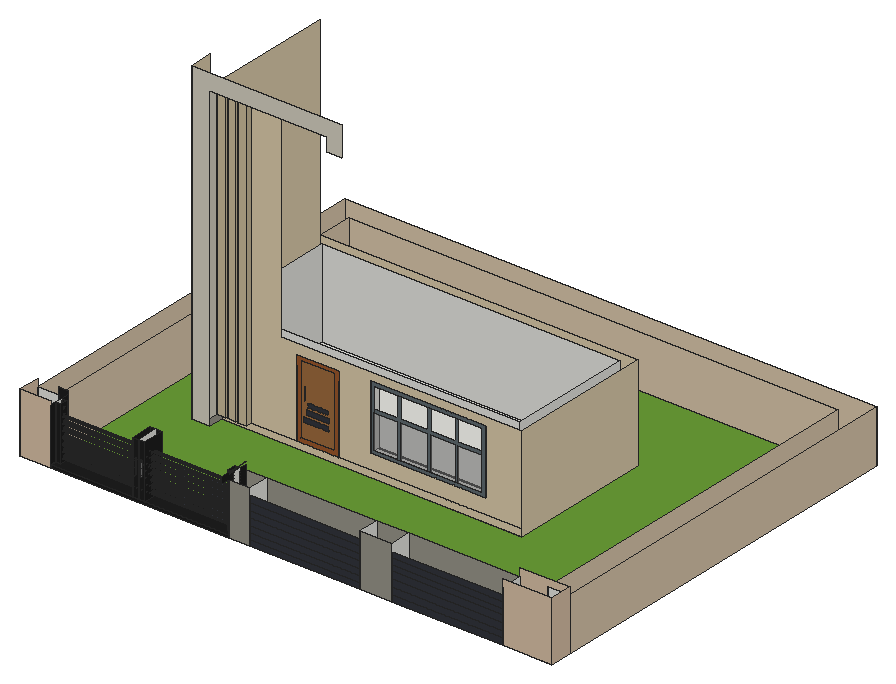
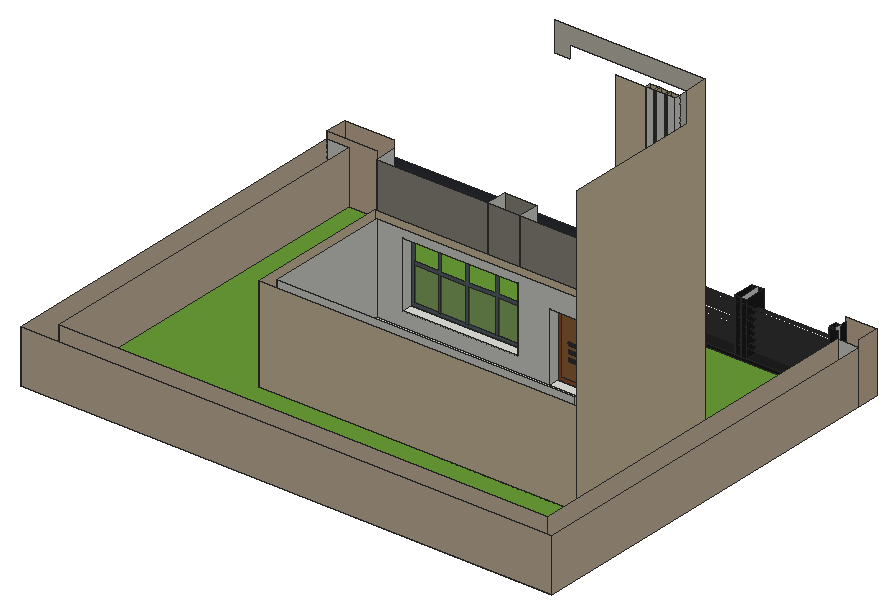
# SketchUp Ruby script. Lengths in inches.
U = 1.inch
M = Sketchup.active_model
def pt(a) = Geom::Point3d.new(a.map { |v| v * U })
def face(e, loops, mat)
  f = e.add_face(loops[0].map { |a| pt(a) })
  loops[1..].each { |l| e.add_face(l.map { |a| pt(a) }).erase! }
  f.material = f.back_material = mat if mat
  f
end
# faces: each face lists its corners as indices into pts; further lists are holes
def faces(e, pts, list, mat = nil) = list.each { |f| face(e, (f[0].is_a?(Array) ? f : [f]).map { |l| l.map { |i| pts[i] } }, mat) }
# xy, xz, yz: faces in a plane at the given z, y or x. An outline is a flat list of corners, or four numbers for a rectangle; further outlines are holes
def ring(l) = l.size == 4 ? [[l[0], l[1]], [l[2], l[1]], [l[2], l[3]], [l[0], l[3]]] : l.each_slice(2).to_a
def flat(e, list, mat, &to3) = list.each { |f| face(e, (f[0].is_a?(Array) ? f : [f]).map { |l| ring(l).map { |u, v| to3.(u, v) } }, mat) }
def xy(e, z, list, mat = nil) = flat(e, list, mat) { |x, y| [x, y, z] }
def xz(e, y, list, mat = nil) = flat(e, list, mat) { |x, z| [x, y, z] }
def yz(e, x, list, mat = nil) = flat(e, list, mat) { |y, z| [x, y, z] }
def lines(e, pts, list) = list.each { |a, b| e.add_line(pt(pts[a]), pt(pts[b])) }
# prism: a flat outline (further loops are holes) pulled along v
def prism(e, loops, v, mat = nil)
  f = face(e, loops, mat); d = Geom::Vector3d.new(v.map { |x| x * U })
  f.pushpull(f.normal.samedirection?(d) ? d.length : -d.length)
end
def box(e, o, s, mat = nil) = prism(e, [[o, [o[0] + s[0], o[1], o[2]], [o[0] + s[0], o[1] + s[1], o[2]], [o[0], o[1] + s[1], o[2]]]], [0, 0, s[2]], mat)
def at(x, y, z, deg = 0) = Geom::Transformation.translation(pt([x, y, z])) * Geom::Transformation.rotation(ORIGIN, Z_AXIS, deg.degrees)
def axes(o, x, y, z) = Geom::Transformation.new([*x, 0, *y, 0, *z, 0, *pt(o).to_a, 1])
def part(name) = M.definitions.add(name)
# library, detail: a bought-in or finely detailed component or shape, given as its bounding box
def library(name, o, s) = part(name).tap { |d| box(d.entities, o, s) }
def detail(e, o, s) = box(e.add_group.entities, o, s)
def put(e, d, t, mat = nil) = e.add_instance(d, t).tap { |i| i.material = mat if mat }
def group(e, t, mat = nil) = e.add_group.tap { |g| g.transformation = t; g.material = mat if mat }.entities
root = M.entities
M.materials.add("[Color M05]").color = [114, 114, 114]
M.materials.add("[Color M08]").color = [30, 30, 30]
M.materials.add("[Field Square Tile]").color = [217, 201, 169]
M.materials.add("[Formica Graystone]").color = [209, 204, 189]
M.materials.add("[Formica Graystone]1").color = [149, 146, 135]
M.materials.add("[Formica Laminate Dark]").color = [50, 53, 60]
M.materials.add("[Formica Laminate Light]").color = [213, 189, 164]
M.materials.add("[Formica Speckled Grey]").color = [94, 105, 111]
M.materials.add("[Grass Dark Green]").color = [106, 157, 55]
M.materials.add("[Quartz Light Brown]").color = [199, 184, 152]
M.materials.add("[Tile Various Tan]").color = [214, 196, 169]
M.materials.add("[Translucent Glass Gray]").color = [128, 128, 128]
M.materials["[Translucent Glass Gray]"].alpha = 0.5
M.materials.add("[Wood Cherry Original]").color = [152, 86, 42]
M.materials.add("[Wood Floor]").color = [155, 105, 61]
xy(root,0,[[0,19.125,41.54,48.44],[41.54,19.125,284.59,48.44],[284.59,19.125,312.84,48.44],[312.84,19.125,463.03,48.44],[463.03,19.125,507.04,48.44],
  [507.04,19.125,658.96,48.44],[658.96,19.125,726.5625,48.44],[0,48.44,0,572.27,726.5625,572.27,726.5625,48.44,697.25,48.44,697.25,542.96,29.31,542.96,29.31,48.44],[92.5625,195.77,92.5625,414.5,526.89,414.5,526.89,216.4,117.23,216.4,117.23,195.77]])
xy(root,0,[[[29.31,48.44,697.25,542.96],[92.5625,195.77,117.23,195.77,117.23,216.4,526.89,216.4,526.89,414.5,92.5625,414.5]]],"[Grass Dark Green]")
xy(root,4.0625,[[153.57,19.125,161.5,48.44],[161.5,19.125,169.43,48.44],[41.54,27.41,48.35,37.79],[277.34,27.41,284.59,37.79]])
xy(root,4.0625,[[41.54,19.125,153.57,19.125,153.57,48.44,41.54,48.44,41.54,37.79,48.35,37.79,48.35,27.41,41.54,27.41],[169.43,19.125,284.59,19.125,284.59,27.41,277.34,27.41,277.34,37.79,284.59,37.79,284.59,48.44,169.43,48.44]],"[Color M08]")
xy(root,9,[[117.23,208.71,128.74,216.4],[131.17,208.71,142.68,216.4],[145.54,208.71,157.05,216.4],[219.375,216.4,276.875,230.18],[106.34,230.18,513.1,400.72]])
xy(root,29.57,[[320.36,216.4,477.43,230.18]])
xz(root,19.125,[[156.51,31.35,159.64,54.1],[163.7,31.35,166.82,54.1]],"[Color M05]")
xz(root,19.125,[[41.54,0,284.59,4.0625],[[153.57,4.0625,161.5,76.75],[156.51,31.35,159.64,54.1]],[[161.5,4.0625,169.43,76.75],[163.7,31.35,166.82,54.1]]],"[Color M08]")
xz(root,19.125,[[284.59,0,312.84,70.6875],[463.03,0,507.04,70.6875]],"[Formica Graystone]1")
xz(root,19.125,[[312.84,0,463.03,7.88],[507.04,0,658.96,8.76],[312.84,7.88,463.03,15.75],[507.04,8.76,658.96,17.52],[312.84,15.75,463.03,24.9375],
  [507.04,17.52,658.96,27.92],[312.84,24.9375,463.03,34.65],[507.04,27.92,658.96,37.26],[312.84,34.65,463.03,42.8],[507.04,37.26,658.96,44.93],
  [312.84,42.8,463.03,52.5625],[507.04,44.93,658.96,53.11],[312.84,52.5625,463.03,61.83],[507.04,53.11,658.96,61.39]],"[Formica Laminate Dark]")
xz(root,19.125,[[0,0,41.54,81.8125],[658.96,0,726.5625,81.8125]],"[Formica Laminate Light]")
xz(root,27.41,[[41.54,4.0625,48.35,76.75],[277.34,4.0625,284.59,76.75]],"[Color M08]")
xz(root,37.79,[[41.54,4.0625,48.35,76.75],[277.34,4.0625,284.59,76.75]],"[Color M08]")
xz(root,48.44,[[0,0,29.31,72],[697.25,0,726.5625,72]])
xz(root,48.44,[[29.31,0,41.54,81.8125],[41.54,0,284.59,4.0625],[153.57,4.0625,161.5,76.75],[161.5,4.0625,169.43,76.75]],"[Color M08]")
xz(root,48.44,[[284.59,0,312.84,70.6875],[312.84,0,463.03,70.6875],[463.03,0,507.04,70.6875],[507.04,0,658.96,70.6875]],"[Formica Graystone]1")
xz(root,48.44,[[658.96,0,658.96,81.8125,726.5625,81.8125,726.5625,72,697.25,72,697.25,0]],"[Formica Laminate Light]")
xz(root,195.77,[[92.5625,0,117.23,0,117.23,409.95,276.68,409.95,276.68,392.375,297.93,392.375,297.93,432.8125,92.5625,432.8125]],"[Formica Graystone]")
xz(root,208.71,[[117.23,9,128.74,409.95],[131.17,9,142.68,409.95],[145.54,9,157.05,409.95]],"[Quartz Light Brown]")
xz(root,216.4,[[117.23,9,128.74,409.95],[131.17,9,142.68,409.95],[145.54,9,157.05,409.95]])
xz(root,216.4,[[117.23,0,526.89,9],[[157.05,9,219.375,9,219.375,114.79,276.875,114.79,276.875,9,526.89,9,526.89,129,198.4375,129,198.4375,409.95,157.05,409.95],[320.36,29.57,477.43,118.13]]],"[Field Square Tile]")
xz(root,216.4,[[128.74,9,131.17,409.95],[142.68,9,145.54,409.95],[235.04,35.8125,263.91,35.8125,263.91,41.5625,229.73,41.5625,229.73,35.9375],[232.91,45.5,263.91,51.25],[235.04,55.375,263.91,61.125]],"[Formica Laminate Dark]")
xz(root,216.4,[[[320.36,29.57,477.43,118.13],[324.95,34.15,472.85,113.55]],[358.29,34.15,361.76,34.15,361.76,80.75,398.73,80.75,398.73,34.15,402.19,34.15,402.19,80.75,436.48,80.75,436.48,34.15,439.94,34.15,439.94,80.75,472.85,80.75,472.85,85.55,439.94,85.55,439.94,113.55,436.48,113.55,436.48,85.55,402.19,85.55,402.19,113.55,398.73,113.55,398.73,85.55,361.76,85.55,361.76,113.55,358.29,113.55,358.29,85.55,324.95,85.55,324.95,80.75,358.29,80.75]],"[Formica Speckled Grey]")
xz(root,216.4,[[324.95,34.15,358.29,80.75],[361.76,34.15,398.73,80.75],[402.19,34.15,436.48,80.75],[439.94,34.15,472.85,80.75]],"[Translucent Glass Gray]")
xz(root,216.4,[[[219.375,9,276.875,114.79],[225.14,14.77,271.11,110.58]]],"[Wood Cherry Original]")
xz(root,216.4,[[[225.14,14.77,271.11,110.58],[235.04,35.8125,229.73,35.9375,229.73,41.5625,263.91,41.5625,263.91,35.8125],[232.91,45.5,263.91,51.25],[235.04,55.375,263.91,61.125],[228.85,61.59,231.85,79.84]]],"[Wood Floor]")
xz(root,230.18,[[[106.34,9,106.34,129,513.1,129,513.1,9,276.875,9,276.875,102.04,219.375,102.04,219.375,9],[320.36,29.57,477.43,118.13]]])
xz(root,400.72,[[106.34,9,513.1,129]])
xz(root,414.5,[[92.5625,0,526.89,129]],"[Field Square Tile]")
xz(root,542.96,[[29.31,0,697.25,72]],"[Tile Various Tan]")
xz(root,572.27,[[0,0,726.5625,72]],"[Tile Various Tan]")
yz(root,0,[[19.125,0,48.44,81.8125]],"[Formica Laminate Light]")
yz(root,0,[[48.44,0,572.27,72]],"[Tile Various Tan]")
yz(root,29.31,[[48.44,0,542.96,72]],"[Tile Various Tan]")
yz(root,41.54,[[19.125,0,48.44,4.0625],[27.41,4.0625,37.79,76.75]])
yz(root,41.54,[[19.125,4.0625,27.41,76.75],[37.79,4.0625,48.44,76.75]],"[Color M08]")
yz(root,48.35,[[33.0625,7.25,32.4,7.34,31.78,7.6,31.25,8,30.84,8.53,30.59,9.15,30.5,9.81,30.59,10.48,30.84,11.1,31.25,11.625,31.78,12.03,32.4,12.29,33.0625,12.38,33.73,12.29,34.34,12.03,34.875,11.625,35.28,11.1,35.54,10.48,35.625,9.81,35.54,9.15,35.28,8.53,34.875,8,34.34,7.6,33.73,7.34],[33.0625,15.81,32.4,15.9,31.78,16.16,31.25,16.57,30.84,17.1,30.59,17.71,30.5,18.38,30.59,19.04,30.84,19.66,31.25,20.1875,31.78,20.6,32.4,20.85,33.0625,20.94,33.73,20.85,34.34,20.6,34.875,20.1875,35.28,19.66,35.54,19.04,35.625,18.38,35.54,17.71,35.28,17.1,34.875,16.57,34.34,16.16,33.73,15.9],[33.0625,23.81,32.4,23.9,31.78,24.16,31.25,24.57,30.84,25.1,30.59,25.71,30.5,26.38,30.59,27.04,30.84,27.66,31.25,28.1875,31.78,28.6,32.4,28.85,33.0625,28.94,33.73,28.85,34.34,28.6,34.875,28.1875,35.28,27.66,35.54,27.04,35.625,26.38,35.54,25.71,35.28,25.1,34.875,24.57,34.34,24.16,33.73,23.9],[33.0625,32.5,32.4,32.59,31.78,32.85,31.25,33.25,30.84,33.78,30.59,34.4,30.5,35.06,30.59,35.73,30.84,36.35,31.25,36.875,31.78,37.28,32.4,37.54,33.0625,37.63,33.73,37.54,34.34,37.28,34.875,36.875,35.28,36.35,35.54,35.73,35.625,35.06,35.54,34.4,35.28,33.78,34.875,33.25,34.34,32.85,33.73,32.59],[33.0625,41.5,32.4,41.59,31.78,41.85,31.25,42.25,30.84,42.78,30.59,43.4,30.5,44.06,30.59,44.73,30.84,45.35,31.25,45.875,31.78,46.28,32.4,46.54,33.0625,46.63,33.73,46.54,34.34,46.28,34.875,45.875,35.28,45.35,35.54,44.73,35.625,44.06,35.54,43.4,35.28,42.78,34.875,42.25,34.34,41.85,33.73,41.59],
  [33.0625,50.06,32.4,50.15,31.78,50.41,31.25,50.82,30.84,51.35,30.59,51.96,30.5,52.63,30.59,53.29,30.84,53.91,31.25,54.4375,31.78,54.85,32.4,55.1,33.0625,55.19,33.73,55.1,34.34,54.85,34.875,54.4375,35.28,53.91,35.54,53.29,35.625,52.63,35.54,51.96,35.28,51.35,34.875,50.82,34.34,50.41,33.73,50.15],[33.0625,58.94,32.4,59.03,31.78,59.28,31.25,59.69,30.84,60.22,30.59,60.84,30.5,61.5,30.59,62.17,30.84,62.78,31.25,63.3125,31.78,63.72,32.4,63.98,33.0625,64.06,33.73,63.98,34.34,63.72,34.875,63.3125,35.28,62.78,35.54,62.17,35.625,61.5,35.54,60.84,35.28,60.22,34.875,59.69,34.34,59.28,33.73,59.03]])
yz(root,48.35,[[[27.41,4.0625,37.79,76.75],[33.0625,67.25,32.4,67.34,31.78,67.6,31.25,68,30.84,68.53,30.59,69.15,30.5,69.81,30.59,70.48,30.84,71.1,31.25,71.625,31.78,72.03,32.4,72.29,33.0625,72.38,33.73,72.29,34.34,72.03,34.875,71.625,35.28,71.1,35.54,70.48,35.625,69.81,35.54,69.15,35.28,68.53,34.875,68,34.34,67.6,33.73,67.34],[33.0625,7.25,32.4,7.34,31.78,7.6,31.25,8,30.84,8.53,30.59,9.15,30.5,9.81,30.59,10.48,30.84,11.1,31.25,11.625,31.78,12.03,32.4,12.29,33.0625,12.38,33.73,12.29,34.34,12.03,34.875,11.625,35.28,11.1,35.54,10.48,35.625,9.81,35.54,9.15,35.28,8.53,34.875,8,34.34,7.6,33.73,7.34],[33.0625,58.94,32.4,59.03,31.78,59.28,31.25,59.69,30.84,60.22,30.59,60.84,30.5,61.5,30.59,62.17,30.84,62.78,31.25,63.3125,31.78,63.72,32.4,63.98,33.0625,64.06,33.73,63.98,34.34,63.72,34.875,63.3125,35.28,62.78,35.54,62.17,35.625,61.5,35.54,60.84,35.28,60.22,34.875,59.69,34.34,59.28,33.73,59.03],[33.0625,15.81,32.4,15.9,31.78,16.16,31.25,16.57,30.84,17.1,30.59,17.71,30.5,18.38,30.59,19.04,30.84,19.66,31.25,20.1875,31.78,20.6,32.4,20.85,33.0625,20.94,33.73,20.85,34.34,20.6,34.875,20.1875,35.28,19.66,35.54,19.04,35.625,18.38,35.54,17.71,35.28,17.1,34.875,16.57,34.34,16.16,33.73,15.9],[33.0625,50.06,32.4,50.15,31.78,50.41,31.25,50.82,30.84,51.35,30.59,51.96,30.5,52.63,30.59,53.29,30.84,53.91,31.25,54.4375,31.78,54.85,32.4,55.1,33.0625,55.19,33.73,55.1,34.34,54.85,34.875,54.4375,35.28,53.91,35.54,53.29,35.625,52.63,35.54,51.96,35.28,51.35,34.875,50.82,34.34,50.41,33.73,50.15],[33.0625,23.81,32.4,23.9,31.78,24.16,31.25,24.57,30.84,25.1,30.59,25.71,30.5,26.38,30.59,27.04,30.84,27.66,31.25,28.1875,31.78,28.6,32.4,28.85,33.0625,28.94,33.73,28.85,34.34,28.6,34.875,28.1875,35.28,27.66,35.54,27.04,35.625,26.38,35.54,25.71,35.28,25.1,34.875,24.57,34.34,24.16,33.73,23.9],[33.0625,41.5,32.4,41.59,31.78,41.85,31.25,42.25,30.84,42.78,30.59,43.4,30.5,44.06,30.59,44.73,30.84,45.35,31.25,45.875,31.78,46.28,32.4,46.54,33.0625,46.63,33.73,46.54,34.34,46.28,34.875,45.875,35.28,45.35,35.54,44.73,35.625,44.06,35.54,43.4,35.28,42.78,34.875,42.25,34.34,41.85,33.73,41.59],[33.0625,32.5,32.4,32.59,31.78,32.85,31.25,33.25,30.84,33.78,30.59,34.4,30.5,35.06,30.59,35.73,30.84,36.35,31.25,36.875,31.78,37.28,32.4,37.54,33.0625,37.63,33.73,37.54,34.34,37.28,34.875,36.875,35.28,36.35,35.54,35.73,35.625,35.06,35.54,34.4,35.28,33.78,34.875,33.25,34.34,32.85,33.73,32.59]]],"[Color M08]")
yz(root,92.5625,[[195.77,0,195.77,432.8125,227.35,432.8125,227.35,392.375,414.5,392.375,414.5,0]],"[Field Square Tile]")
yz(root,106.34,[[230.18,9,400.72,129]])
yz(root,117.23,[[208.71,9,216.4,409.95]])
yz(root,117.23,[[195.77,9,208.71,409.95]],"[Formica Graystone]")
yz(root,117.23,[[195.77,0,216.4,9]],"[Formica Graystone]1")
yz(root,128.74,[[208.71,9,216.4,409.95]],"[Quartz Light Brown]")
yz(root,131.17,[[208.71,9,216.4,409.95]],"[Quartz Light Brown]")
yz(root,142.68,[[208.71,9,216.4,409.95]],"[Quartz Light Brown]")
yz(root,145.54,[[208.71,9,216.4,409.95]],"[Quartz Light Brown]")
yz(root,153.57,[[19.125,4.0625,48.44,76.75]],"[Color M08]")
yz(root,157.05,[[208.71,9,216.4,409.95]],"[Quartz Light Brown]")
yz(root,161.5,[[19.125,4.0625,48.44,76.75]])
yz(root,169.43,[[19.125,4.0625,48.44,76.75]],"[Color M08]")
yz(root,219.375,[[216.4,9,230.18,102.04]])
yz(root,276.875,[[216.4,9,230.18,102.04]])
yz(root,277.34,[[[27.41,4.0625,37.79,76.75],[33.0625,67.25,33.73,67.34,34.34,67.6,34.875,68,35.28,68.53,35.54,69.15,35.625,69.81,35.54,70.48,35.28,71.1,34.875,71.625,34.34,72.03,33.73,72.29,33.0625,72.38,32.4,72.29,31.78,72.03,31.25,71.625,30.84,71.1,30.59,70.48,30.5,69.81,30.59,69.15,30.84,68.53,31.25,68,31.78,67.6,32.4,67.34],[33.0625,58.94,33.73,59.03,34.34,59.28,34.875,59.69,35.28,60.22,35.54,60.84,35.625,61.5,35.54,62.17,35.28,62.78,34.875,63.3125,34.34,63.72,33.73,63.98,33.0625,64.06,32.4,63.98,31.78,63.72,31.25,63.3125,30.84,62.78,30.59,62.17,30.5,61.5,30.59,60.84,30.84,60.22,31.25,59.69,31.78,59.28,32.4,59.03],[33.0625,50.06,33.73,50.15,34.34,50.41,34.875,50.82,35.28,51.35,35.54,51.96,35.625,52.63,35.54,53.29,35.28,53.91,34.875,54.4375,34.34,54.85,33.73,55.1,33.0625,55.19,32.4,55.1,31.78,54.85,31.25,54.4375,30.84,53.91,30.59,53.29,30.5,52.63,30.59,51.96,30.84,51.35,31.25,50.82,31.78,50.41,32.4,50.15],[33.0625,41.5,33.73,41.59,34.34,41.85,34.875,42.25,35.28,42.78,35.54,43.4,35.625,44.06,35.54,44.73,35.28,45.35,34.875,45.875,34.34,46.28,33.73,46.54,33.0625,46.63,32.4,46.54,31.78,46.28,31.25,45.875,30.84,45.35,30.59,44.73,30.5,44.06,30.59,43.4,30.84,42.78,31.25,42.25,31.78,41.85,32.4,41.59],[33.0625,32.5,33.73,32.59,34.34,32.85,34.875,33.25,35.28,33.78,35.54,34.4,35.625,35.06,35.54,35.73,35.28,36.35,34.875,36.875,34.34,37.28,33.73,37.54,33.0625,37.63,32.4,37.54,31.78,37.28,31.25,36.875,30.84,36.35,30.59,35.73,30.5,35.06,30.59,34.4,30.84,33.78,31.25,33.25,31.78,32.85,32.4,32.59],[33.0625,23.81,33.73,23.9,34.34,24.16,34.875,24.57,35.28,25.1,35.54,25.71,35.625,26.38,35.54,27.04,35.28,27.66,34.875,28.1875,34.34,28.6,33.73,28.85,33.0625,28.94,32.4,28.85,31.78,28.6,31.25,28.1875,30.84,27.66,30.59,27.04,30.5,26.38,30.59,25.71,30.84,25.1,31.25,24.57,31.78,24.16,32.4,23.9],[33.0625,15.81,33.73,15.9,34.34,16.16,34.875,16.57,35.28,17.1,35.54,17.71,35.625,18.38,35.54,19.04,35.28,19.66,34.875,20.1875,34.34,20.6,33.73,20.85,33.0625,20.94,32.4,20.85,31.78,20.6,31.25,20.1875,30.84,19.66,30.59,19.04,30.5,18.38,30.59,17.71,30.84,17.1,31.25,16.57,31.78,16.16,32.4,15.9],[33.0625,7.25,33.73,7.34,34.34,7.6,34.875,8,35.28,8.53,35.54,9.15,35.625,9.81,35.54,10.48,35.28,11.1,34.875,11.625,34.34,12.03,33.73,12.29,33.0625,12.38,32.4,12.29,31.78,12.03,31.25,11.625,30.84,11.1,30.59,10.48,30.5,9.81,30.59,9.15,30.84,8.53,31.25,8,31.78,7.6,32.4,7.34]]],"[Color M08]")
yz(root,284.59,[[19.125,0,48.44,4.0625],[27.41,4.0625,37.79,76.75]])
yz(root,284.59,[[19.125,4.0625,19.125,70.6875,8,70.6875,8,80,48.44,80,48.44,79.91,19.125,79.91,19.125,76.75,27.41,76.75,27.41,4.0625],[37.79,4.0625,48.44,76.75]],"[Color M08]")
yz(root,312.84,[[19.125,0,48.44,70.6875]])
yz(root,320.36,[[216.4,29.57,230.18,118.13]])
yz(root,463.03,[[19.125,0,48.44,70.6875]])
yz(root,477.43,[[216.4,29.57,230.18,118.13]])
yz(root,507.04,[[19.125,0,48.44,70.6875]])
yz(root,513.1,[[230.18,9,400.72,129]])
yz(root,526.89,[[216.4,0,414.5,129]],"[Field Square Tile]")
yz(root,658.96,[[19.125,0,48.44,70.6875]])
yz(root,697.25,[[48.44,0,542.96,72]],"[Tile Various Tan]")
yz(root,726.5625,[[19.125,0,48.44,81.8125]],"[Formica Laminate Light]")
yz(root,726.5625,[[48.44,0,572.27,72]],"[Tile Various Tan]")
p = [[48.35,31.78,7.6],[48.35,32.4,7.34],[277.34,32.4,7.34],[277.34,31.78,7.6],[48.35,33.0625,7.25],[277.34,33.0625,7.25],
  [48.35,33.73,7.34],[277.34,33.73,7.34],[48.35,34.34,7.6],[277.34,34.34,7.6],[48.35,31.25,8],[277.34,31.25,8],
  [48.35,34.875,8],[277.34,34.875,8],[48.35,30.84,8.53],[277.34,30.84,8.53],[48.35,35.28,8.53],[277.34,35.28,8.53],
  [48.35,30.59,9.15],[277.34,30.59,9.15],[48.35,35.54,9.15],[277.34,35.54,9.15],[48.35,30.5,9.81],[277.34,30.5,9.81],
  [48.35,35.625,9.81],[277.34,35.625,9.81],[48.35,30.59,10.48],[277.34,30.59,10.48],[48.35,35.54,10.48],[277.34,35.54,10.48],
  [48.35,30.84,11.1],[277.34,30.84,11.1],[48.35,35.28,11.1],[277.34,35.28,11.1],[48.35,31.25,11.625],[277.34,31.25,11.625],
  [48.35,34.875,11.625],[277.34,34.875,11.625],[48.35,31.78,12.03],[277.34,31.78,12.03],[48.35,34.34,12.03],[277.34,34.34,12.03],
  [48.35,32.4,12.29],[277.34,32.4,12.29],[48.35,33.73,12.29],[277.34,33.73,12.29],[48.35,33.0625,12.38],[277.34,33.0625,12.38],
  [48.35,32.4,15.9],[48.35,33.0625,15.81],[277.34,33.0625,15.81],[277.34,32.4,15.9],[48.35,33.73,15.9],[277.34,33.73,15.9],
  [48.35,31.78,16.16],[277.34,31.78,16.16],[48.35,34.34,16.16],[277.34,34.34,16.16],[48.35,31.25,16.57],[277.34,31.25,16.57],
  [48.35,34.875,16.57],[277.34,34.875,16.57],[48.35,30.84,17.1],[277.34,30.84,17.1],[48.35,35.28,17.1],[277.34,35.28,17.1],
  [48.35,30.59,17.71],[277.34,30.59,17.71],[48.35,35.54,17.71],[277.34,35.54,17.71],[48.35,30.5,18.38],[277.34,30.5,18.38],
  [48.35,35.625,18.38],[277.34,35.625,18.38],[48.35,30.59,19.04],[277.34,30.59,19.04],[48.35,35.54,19.04],[277.34,35.54,19.04],
  [48.35,30.84,19.66],[277.34,30.84,19.66],[48.35,35.28,19.66],[277.34,35.28,19.66],[48.35,31.25,20.1875],[277.34,31.25,20.1875],
  [48.35,34.875,20.1875],[277.34,34.875,20.1875],[48.35,31.78,20.6],[277.34,31.78,20.6],[48.35,34.34,20.6],[277.34,34.34,20.6],
  [48.35,32.4,20.85],[277.34,32.4,20.85],[48.35,33.73,20.85],[277.34,33.73,20.85],[48.35,33.0625,20.94],[277.34,33.0625,20.94],
  [48.35,32.4,23.9],[48.35,33.0625,23.81],[277.34,33.0625,23.81],[277.34,32.4,23.9],[48.35,33.73,23.9],[277.34,33.73,23.9],
  [48.35,31.78,24.16],[277.34,31.78,24.16],[48.35,34.34,24.16],[277.34,34.34,24.16],[48.35,31.25,24.57],[277.34,31.25,24.57],
  [48.35,34.875,24.57],[277.34,34.875,24.57],[48.35,30.84,25.1],[277.34,30.84,25.1],[48.35,35.28,25.1],[277.34,35.28,25.1],
  [48.35,30.59,25.71],[277.34,30.59,25.71],[48.35,35.54,25.71],[277.34,35.54,25.71],[48.35,30.5,26.38],[277.34,30.5,26.38],
  [48.35,35.625,26.38],[277.34,35.625,26.38],[48.35,30.59,27.04],[277.34,30.59,27.04],[48.35,35.54,27.04],[277.34,35.54,27.04],
  [48.35,30.84,27.66],[277.34,30.84,27.66],[48.35,35.28,27.66],[277.34,35.28,27.66],[48.35,31.25,28.1875],[277.34,31.25,28.1875],
  [48.35,34.875,28.1875],[277.34,34.875,28.1875],[48.35,31.78,28.6],[277.34,31.78,28.6],[48.35,34.34,28.6],[277.34,34.34,28.6],
  [48.35,32.4,28.85],[277.34,32.4,28.85],[48.35,33.73,28.85],[277.34,33.73,28.85],[48.35,33.0625,28.94],[277.34,33.0625,28.94],
  [48.35,32.4,32.59],[48.35,33.0625,32.5],[277.34,33.0625,32.5],[277.34,32.4,32.59],[48.35,33.73,32.59],[277.34,33.73,32.59],
  [48.35,31.78,32.85],[277.34,31.78,32.85],[48.35,34.34,32.85],[277.34,34.34,32.85],[48.35,31.25,33.25],[277.34,31.25,33.25],
  [48.35,34.875,33.25],[277.34,34.875,33.25],[48.35,30.84,33.78],[277.34,30.84,33.78],[48.35,35.28,33.78],[277.34,35.28,33.78],
  [48.35,30.59,34.4],[277.34,30.59,34.4],[48.35,35.54,34.4],[277.34,35.54,34.4],[48.35,30.5,35.06],[277.34,30.5,35.06],
  [48.35,35.625,35.06],[277.34,35.625,35.06],[48.35,30.59,35.73],[277.34,30.59,35.73],[48.35,35.54,35.73],[277.34,35.54,35.73],
  [48.35,30.84,36.35],[277.34,30.84,36.35],[48.35,35.28,36.35],[277.34,35.28,36.35],[48.35,31.25,36.875],[277.34,31.25,36.875],
  [48.35,34.875,36.875],[277.34,34.875,36.875],[48.35,31.78,37.28],[277.34,31.78,37.28],[48.35,34.34,37.28],[277.34,34.34,37.28],
  [48.35,32.4,37.54],[277.34,32.4,37.54],[48.35,33.73,37.54],[277.34,33.73,37.54],[48.35,33.0625,37.63],[277.34,33.0625,37.63],
  [48.35,32.4,41.59],[48.35,33.0625,41.5],[277.34,33.0625,41.5],[277.34,32.4,41.59],[48.35,33.73,41.59],[277.34,33.73,41.59],
  [48.35,31.78,41.85],[277.34,31.78,41.85],[48.35,34.34,41.85],[277.34,34.34,41.85],[48.35,31.25,42.25],[277.34,31.25,42.25],
  [48.35,34.875,42.25],[277.34,34.875,42.25],[48.35,30.84,42.78],[277.34,30.84,42.78],[48.35,35.28,42.78],[277.34,35.28,42.78],
  [48.35,30.59,43.4],[277.34,30.59,43.4],[48.35,35.54,43.4],[277.34,35.54,43.4],[48.35,30.5,44.06],[277.34,30.5,44.06],
  [48.35,35.625,44.06],[277.34,35.625,44.06],[48.35,30.59,44.73],[277.34,30.59,44.73],[48.35,35.54,44.73],[277.34,35.54,44.73],
  [48.35,30.84,45.35],[277.34,30.84,45.35],[48.35,35.28,45.35],[277.34,35.28,45.35],[48.35,31.25,45.875],[277.34,31.25,45.875],
  [48.35,34.875,45.875],[277.34,34.875,45.875],[48.35,31.78,46.28],[277.34,31.78,46.28],[48.35,34.34,46.28],[277.34,34.34,46.28],
  [48.35,32.4,46.54],[277.34,32.4,46.54],[48.35,33.73,46.54],[277.34,33.73,46.54],[48.35,33.0625,46.63],[277.34,33.0625,46.63],
  [48.35,32.4,50.15],[48.35,33.0625,50.06],[277.34,33.0625,50.06],[277.34,32.4,50.15],[48.35,33.73,50.15],[277.34,33.73,50.15],
  [48.35,31.78,50.41],[277.34,31.78,50.41],[48.35,34.34,50.41],[277.34,34.34,50.41],[48.35,31.25,50.82],[277.34,31.25,50.82],
  [48.35,34.875,50.82],[277.34,34.875,50.82],[48.35,30.84,51.35],[277.34,30.84,51.35],[48.35,35.28,51.35],[277.34,35.28,51.35],
  [48.35,30.59,51.96],[277.34,30.59,51.96],[48.35,35.54,51.96],[277.34,35.54,51.96],[48.35,30.5,52.63],[277.34,30.5,52.63],
  [48.35,35.625,52.63],[277.34,35.625,52.63],[48.35,30.59,53.29],[277.34,30.59,53.29],[48.35,35.54,53.29],[277.34,35.54,53.29],
  [48.35,30.84,53.91],[277.34,30.84,53.91],[48.35,35.28,53.91],[277.34,35.28,53.91],[48.35,31.25,54.4375],[277.34,31.25,54.4375],
  [48.35,34.875,54.4375],[277.34,34.875,54.4375],[48.35,31.78,54.85],[277.34,31.78,54.85],[48.35,34.34,54.85],[277.34,34.34,54.85],
  [48.35,32.4,55.1],[277.34,32.4,55.1],[48.35,33.73,55.1],[277.34,33.73,55.1],[48.35,33.0625,55.19],[277.34,33.0625,55.19],
  [48.35,32.4,59.03],[48.35,33.0625,58.94],[277.34,33.0625,58.94],[277.34,32.4,59.03],[48.35,33.73,59.03],[277.34,33.73,59.03],
  [48.35,31.78,59.28],[277.34,31.78,59.28],[48.35,34.34,59.28],[277.34,34.34,59.28],[48.35,31.25,59.69],[277.34,31.25,59.69],
  [48.35,34.875,59.69],[277.34,34.875,59.69],[48.35,30.84,60.22],[277.34,30.84,60.22],[48.35,35.28,60.22],[277.34,35.28,60.22],
  [106.34,230.18,9],[92.5625,230.18,9]]
faces(root,p,[[0,1,2,3],[1,4,5,2],[4,6,7,5],[6,8,9,7],[10,0,3,11],[8,12,13,9],[14,10,11,15],[12,16,17,13],
  [18,14,15,19],[16,20,21,17],[22,18,19,23],[20,24,25,21],[26,22,23,27],[24,28,29,25],[30,26,27,31],[28,32,33,29],
  [34,30,31,35],[32,36,37,33],[38,34,35,39],[36,40,41,37],[42,38,39,43],[40,44,45,41],[46,42,43,47],[44,46,47,45],
  [48,49,50,51],[49,52,53,50],[54,48,51,55],[52,56,57,53],[58,54,55,59],[56,60,61,57],[62,58,59,63],[60,64,65,61],
  [66,62,63,67],[64,68,69,65],[70,66,67,71],[68,72,73,69],[74,70,71,75],[72,76,77,73],[78,74,75,79],[76,80,81,77],
  [82,78,79,83],[80,84,85,81],[86,82,83,87],[84,88,89,85],[90,86,87,91],[88,92,93,89],[94,90,91,95],[92,94,95,93],
  [96,97,98,99],[97,100,101,98],[102,96,99,103],[100,104,105,101],[106,102,103,107],[104,108,109,105],[110,106,107,111],[108,112,113,109],
  [114,110,111,115],[112,116,117,113],[118,114,115,119],[116,120,121,117],[122,118,119,123],[120,124,125,121],[126,122,123,127],[124,128,129,125],
  [130,126,127,131],[128,132,133,129],[134,130,131,135],[132,136,137,133],[138,134,135,139],[136,140,141,137],[142,138,139,143],[140,142,143,141],
  [144,145,146,147],[145,148,149,146],[150,144,147,151],[148,152,153,149],[154,150,151,155],[152,156,157,153],[158,154,155,159],[156,160,161,157],
  [162,158,159,163],[160,164,165,161],[166,162,163,167],[164,168,169,165],[170,166,167,171],[168,172,173,169],[174,170,171,175],[172,176,177,173],
  [178,174,175,179],[176,180,181,177],[182,178,179,183],[180,184,185,181],[186,182,183,187],[184,188,189,185],[190,186,187,191],[188,190,191,189],
  [192,193,194,195],[193,196,197,194],[198,192,195,199],[196,200,201,197],[202,198,199,203],[200,204,205,201],[206,202,203,207],[204,208,209,205],
  [210,206,207,211],[208,212,213,209],[214,210,211,215],[212,216,217,213],[218,214,215,219],[216,220,221,217],[222,218,219,223],[220,224,225,221],
  [226,222,223,227],[224,228,229,225],[230,226,227,231],[228,232,233,229],[234,230,231,235],[232,236,237,233],[238,234,235,239],[236,238,239,237],
  [240,241,242,243],[241,244,245,242],[246,240,243,247],[244,248,249,245],[250,246,247,251],[248,252,253,249],[254,250,251,255],[252,256,257,253],
  [258,254,255,259],[256,260,261,257],[262,258,259,263],[260,264,265,261],[266,262,263,267],[264,268,269,265],[270,266,267,271],[268,272,273,269],
  [274,270,271,275],[272,276,277,273],[278,274,275,279],[276,280,281,277],[282,278,279,283],[280,284,285,281],[286,282,283,287],[284,286,287,285],
  [288,289,290,291],[289,292,293,290],[294,288,291,295],[292,296,297,293],[298,294,295,299],[296,300,301,297],[302,298,299,303],[300,304,305,301]],"[Formica Laminate Dark]")
lines(root,p,[[306,307]])
